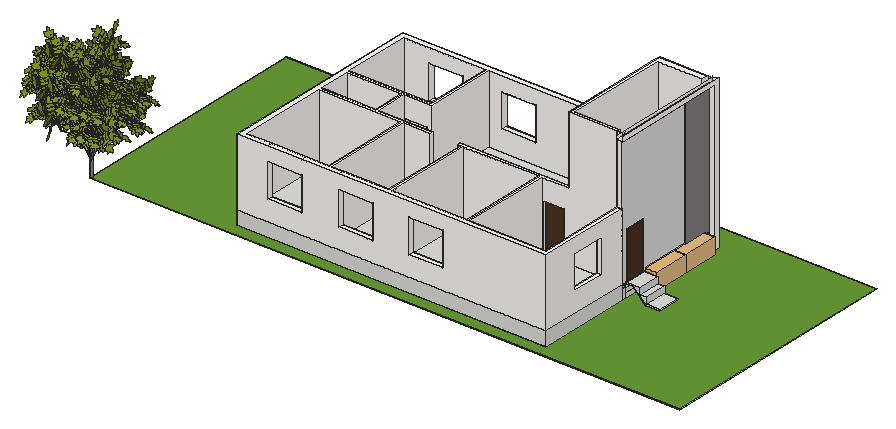
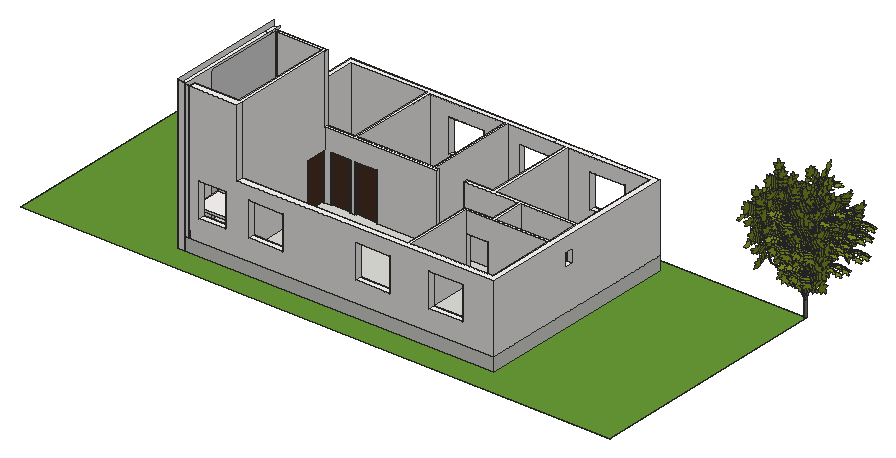
# SketchUp Ruby script. Lengths in inches.
U = 1.inch
M = Sketchup.active_model
def pt(a) = Geom::Point3d.new(a.map { |v| v * U })
def face(e, loops, mat)
  f = e.add_face(loops[0].map { |a| pt(a) })
  loops[1..].each { |l| e.add_face(l.map { |a| pt(a) }).erase! }
  f.material = f.back_material = mat if mat
  f
end
# faces: each face lists its corners as indices into pts; further lists are holes
def faces(e, pts, list, mat = nil) = list.each { |f| face(e, (f[0].is_a?(Array) ? f : [f]).map { |l| l.map { |i| pts[i] } }, mat) }
# xy, xz, yz: faces in a plane at the given z, y or x. An outline is a flat list of corners, or four numbers for a rectangle; further outlines are holes
def ring(l) = l.size == 4 ? [[l[0], l[1]], [l[2], l[1]], [l[2], l[3]], [l[0], l[3]]] : l.each_slice(2).to_a
def flat(e, list, mat, &to3) = list.each { |f| face(e, (f[0].is_a?(Array) ? f : [f]).map { |l| ring(l).map { |u, v| to3.(u, v) } }, mat) }
def xy(e, z, list, mat = nil) = flat(e, list, mat) { |x, y| [x, y, z] }
def xz(e, y, list, mat = nil) = flat(e, list, mat) { |x, z| [x, y, z] }
def yz(e, x, list, mat = nil) = flat(e, list, mat) { |y, z| [x, y, z] }
def lines(e, pts, list) = list.each { |a, b| e.add_line(pt(pts[a]), pt(pts[b])) }
# prism: a flat outline (further loops are holes) pulled along v
def prism(e, loops, v, mat = nil)
  f = face(e, loops, mat); d = Geom::Vector3d.new(v.map { |x| x * U })
  f.pushpull(f.normal.samedirection?(d) ? d.length : -d.length)
end
def box(e, o, s, mat = nil) = prism(e, [[o, [o[0] + s[0], o[1], o[2]], [o[0] + s[0], o[1] + s[1], o[2]], [o[0], o[1] + s[1], o[2]]]], [0, 0, s[2]], mat)
def at(x, y, z, deg = 0) = Geom::Transformation.translation(pt([x, y, z])) * Geom::Transformation.rotation(ORIGIN, Z_AXIS, deg.degrees)
def axes(o, x, y, z) = Geom::Transformation.new([*x, 0, *y, 0, *z, 0, *pt(o).to_a, 1])
def part(name) = M.definitions.add(name)
# library, detail: a bought-in or finely detailed component or shape, given as its bounding box
def library(name, o, s) = part(name).tap { |d| box(d.entities, o, s) }
def detail(e, o, s) = box(e.add_group.entities, o, s)
def put(e, d, t, mat = nil) = e.add_instance(d, t).tap { |i| i.material = mat if mat }
def group(e, t, mat = nil) = e.add_group.tap { |g| g.transformation = t; g.material = mat if mat }.entities
root = M.entities
M.materials.add("3D66_SU_1574822641685_001").color = [135, 150, 36]
M.materials.add("3D66_SU_1574822641883_002").color = [178, 165, 164]
M.materials.add("3D66_SU_1574822642012_003").color = [128, 125, 127]
M.materials.add("Polis06_194").color = [79, 50, 36]
M.materials.add("[0010_Snow]").color = [255, 250, 250]
M.materials.add("[Brick Tumbled]").color = [135, 132, 132]
M.materials.add("[Color M01]").color = [226, 226, 226]
M.materials.add("[Grass Dark Green]").color = [106, 157, 55]
c1 = part("Group16\#1")
prism(c1.entities,[[[640.68,60.08,-12.85],[640.68,60.08,-11.85],[640.68,36.46,-11.85],[640.68,36.46,-17.72],[640.68,24.64,-17.72],[640.68,24.64,-23.6],[640.68,1.02,-23.6],[640.68,1.02,-24.6],[640.68,24.88,-24.6],[640.68,48.5,-12.85]]],[-39.375,0,0])
c2 = part("Group7\#1")
p = [[645.1,1113.3,118],[645.1,1115.23,118],[645.1,1197.92,159.125],[645.1,1235.36,159.125],[723.92,1235.36,159.125],[723.92,1197.92,159.125],
  [723.92,1103.42,206.125],[723.92,1091.61,206.125],[680.6,1113.3,118],[680.6,1115.23,118],[680.6,1197.92,159.125],[680.6,1199.86,159.125],
  [688.42,1199.86,159.125],[688.42,1197.92,159.125],[688.42,1103.42,206.125],[688.42,1091.61,206.125]]
lines(c2.entities,p,[[0,1],[1,2],[2,3],[3,4],[4,5],[5,6],[6,7],[8,9],[9,10],[10,11],[11,12],[12,13],
  [13,14],[14,15]])
c3 = part("Group6\#1")
xy(c3.entities,114.0625,[[643.17,1127.05,682.54,1127.97]])
xy(c3.entities,118,[[643.17,1115.23,682.54,1127.05]])
xy(c3.entities,123.875,[[643.17,1127.05,682.54,1138.86]])
xy(c3.entities,129.75,[[643.17,1138.86,682.54,1150.67]])
xy(c3.entities,135.625,[[643.17,1150.67,682.54,1162.48]])
xy(c3.entities,141.5,[[643.17,1162.48,682.54,1174.3]])
xy(c3.entities,147.375,[[643.17,1174.3,682.54,1186.11]])
xy(c3.entities,153.25,[[643.17,1186.11,682.54,1197.92]])
xy(c3.entities,155.1875,[[686.48,1185.18,686.48,1197.92,682.54,1197.92,682.54,1210.66,643.17,1210.66,643.17,1237.3,725.85,1237.3,725.85,1185.18]])
xy(c3.entities,159.125,[[686.48,1186.11,725.85,1186.11,725.85,1237.3,643.17,1237.3,643.17,1197.92,686.48,1197.92]])
xy(c3.entities,165,[[686.48,1174.3,725.85,1186.11]])
xy(c3.entities,170.875,[[686.48,1162.48,725.85,1174.3]])
xy(c3.entities,176.75,[[686.48,1150.67,725.85,1162.48]])
xy(c3.entities,182.625,[[686.48,1138.86,725.85,1150.67]])
xy(c3.entities,188.5,[[686.48,1127.05,725.85,1138.86]])
xy(c3.entities,194.375,[[686.48,1115.23,725.85,1127.05]])
xy(c3.entities,200.25,[[686.48,1103.42,725.85,1115.23]])
xy(c3.entities,206.125,[[686.48,1091.61,725.85,1103.42]])
xz(c3.entities,1103.42,[[686.48,200.25,725.85,206.125]])
xz(c3.entities,1115.23,[[686.48,194.375,725.85,200.25]])
xz(c3.entities,1127.05,[[643.17,118,682.54,123.875],[686.48,188.5,725.85,194.375]])
xz(c3.entities,1138.86,[[643.17,123.875,682.54,129.75],[686.48,182.625,725.85,188.5]])
xz(c3.entities,1150.67,[[643.17,129.75,682.54,135.625],[686.48,176.75,725.85,182.625]])
xz(c3.entities,1162.48,[[643.17,135.625,682.54,141.5],[686.48,170.875,725.85,176.75]])
xz(c3.entities,1174.3,[[643.17,141.5,682.54,147.375],[686.48,165,725.85,170.875]])
xz(c3.entities,1186.11,[[643.17,147.375,682.54,153.25],[686.48,159.125,725.85,165]])
xz(c3.entities,1197.92,[[643.17,153.25,682.54,159.125],[682.54,155.1875,686.48,159.125]])
xz(c3.entities,1237.3,[[643.17,155.1875,725.85,159.125]])
yz(c3.entities,643.17,[[1127.05,114.0625,1127.05,123.875,1138.86,123.875,1138.86,129.75,1150.67,129.75,1150.67,135.625,1162.48,135.625,1162.48,141.5,1174.3,141.5,1174.3,147.375,1186.11,147.375,1186.11,153.25,1197.92,153.25,1197.92,159.125,1237.3,159.125,1237.3,155.1875,1210.66,155.1875,1127.97,114.0625]])
yz(c3.entities,682.54,[[1127.05,114.0625,1127.97,114.0625,1210.66,155.1875,1197.92,155.1875,1197.92,153.25,1186.11,153.25,1186.11,147.375,1174.3,147.375,1174.3,141.5,1162.48,141.5,1162.48,135.625,1150.67,135.625,1150.67,129.75,1138.86,129.75,1138.86,123.875,1127.05,123.875]])
yz(c3.entities,686.48,[[1185.18,155.1875,1090.68,202.1875,1091.61,202.1875,1091.61,206.125,1103.42,206.125,1103.42,200.25,1115.23,200.25,1115.23,194.375,1127.05,194.375,1127.05,188.5,1138.86,188.5,1138.86,182.625,1150.67,182.625,1150.67,176.75,1162.48,176.75,1162.48,170.875,1174.3,170.875,1174.3,165,1186.11,165,1186.11,159.125,1197.92,159.125,1197.92,155.1875]])
yz(c3.entities,725.85,[[1185.18,155.1875,1237.3,155.1875,1237.3,159.125,1186.11,159.125,1186.11,165,1174.3,165,1174.3,170.875,1162.48,170.875,1162.48,176.75,1150.67,176.75,1150.67,182.625,1138.86,182.625,1138.86,188.5,1127.05,188.5,1127.05,194.375,1115.23,194.375,1115.23,200.25,1103.42,200.25,1103.42,206.125,1091.61,206.125,1091.61,202.1875,1090.68,202.1875]])
p = [[643.17,1127.97,114.0625],[643.17,1210.66,155.1875],[682.54,1210.66,155.1875],[682.54,1127.97,114.0625],[725.85,1185.18,155.1875],[725.85,1090.68,202.1875],
  [686.48,1090.68,202.1875],[686.48,1185.18,155.1875]]
faces(c3.entities,p,[[0,1,2,3],[4,5,6,7]])
put(c3.entities,c2,at(0,0,39.375))
c4 = library("Group8",[-183.25,9.15,0],[25.91,56.79,43.93])
c5 = part("Group\#3")
xy(c5.entities,0,[[0,0,4.72,1.18],[0,34.25,4.72,35.43]],"Polis06_194")
xy(c5.entities,85.26,[[0,1.18,4.72,34.25]],"Polis06_194")
xy(c5.entities,86.61,[[0,0,4.72,35.43]],"Polis06_194")
xz(c5.entities,0,[[0,0,4.72,86.61]],"Polis06_194")
xz(c5.entities,1.18,[[0,0,2.36,85.26],[2.36,0,4.72,85.26]],"Polis06_194")
xz(c5.entities,34.25,[[0,0,4.72,85.26]],"Polis06_194")
xz(c5.entities,35.43,[[0,0,4.72,86.61]],"Polis06_194")
yz(c5.entities,0,[[0,0,1.18,86.61],[34.25,0,35.43,86.61],[1.18,85.26,34.25,86.61]],"Polis06_194")
yz(c5.entities,2.36,[[1.18,0,34.25,0,34.25,85.21,1.18,85.26]],"Polis06_194")
yz(c5.entities,4.72,[[0,0,1.18,86.61],[34.25,0,35.43,86.61],[1.18,85.26,34.25,86.61]],"Polis06_194")
c6 = part("rama-acacia")
p = [[-13.8,1.01,-1.08],[-13.61,0.91,-1.04],[-13.61,0.85,-1.06],[-14.07,0.85,-1.21],[-15.17,0.86,-1.58],[-15.95,0.92,-1.83],
  [-16.01,1,-1.83],[-16.01,1.17,-1.78],[-16.07,1.93,-1.6],[-16.4,2.73,-1.5],[-16.65,3.06,-1.5],[-17.13,4.01,-1.41],
  [-17.78,4.7,-1.44],[-18.28,5.07,-1.51],[-18.57,5.18,-1.58],[-18.91,5.47,-1.62],[-19.07,5.48,-1.67],[-19.35,5.61,-1.73],
  [-19.51,5.64,-1.78],[-19.38,5.57,-1.75],[-19.33,5.5,-1.75],[-19.31,5.23,-1.82],[-19.38,5.08,-1.89],[-19.41,4.84,-1.96],
  [-19.36,4.59,-2.01],[-19.43,4.55,-2.04],[-19.36,4.15,-2.125],[-19.21,3.7,-2.19],[-18.875,3.1,-2.24],[-18.61,2.78,-2.24],
  [-17.83,2.19,-2.13],[-17.4375,1.85,-2.09],[-17.04,1.49,-2.05],[-16.61,1.24,-1.97],[-16.17,1.0625,-1.87],[-16.06,0.95,-1.86],
  [-16.06,0.91,-1.87],[-16.32,0.9,-1.96],[-16.7,0.88,-2.1],[-17.05,0.91,-2.21],[-17.61,1.15,-2.33],[-18.06,1.29,-2.45],
  [-18.88,1.53,-2.67],[-20.25,1.46,-3.15],[-20.59,1.49,-3.26],[-20.79,1.37,-3.36],[-21.08,1.2,-3.5],[-21.28,1.22,-3.5625],
  [-21.48,0.94,-3.71],[-21.79,0.5,-3.93],[-22.02,0.17,-4.1],[-22.11,0.05,-4.16],[-22.21,-0.02,-4.21],[-22.375,-0.05,-4.28],
  [-22.375,-0.07,-4.28],[-22.18,-0.09,-4.22],[-22.11,-0.07,-4.19],[-21.78,-0.1,-4.09],[-21.6,-0.18,-4.05],[-21.52,-0.27,-4.04],
  [-21.33,-0.33,-4],[-20.94,-0.54,-3.92],[-20.6875,-0.63,-3.86],[-20.54,-0.68,-3.82],[-20.42,-0.67,-3.78],[-20.09,-0.46,-3.61],
  [-19.8,-0.24,-3.45],[-19.21,-0.02,-3.19],[-18.48,0.08,-2.92],[-17.72,0.38,-2.58],[-17.4,0.5,-2.4375],[-16.93,0.75,-2.21],
  [-16.78,0.8,-2.15],[-16.1,0.83,-1.91],[-16.0625,0.81,-1.9],[-16.08,0.77,-1.91],[-16.27,0.72,-1.99],[-16.88,0.39,-2.29],
  [-17.1875,0.15,-2.46],[-17.27,0.02,-2.52],[-17.94,-0.52,-2.89],[-17.94,-0.59,-2.91],[-18.08,-0.68,-2.99],[-18.13,-0.86,-3.05],
  [-18.56,-1.55,-3.38],[-18.71,-2.11,-3.58],[-18.79,-2.61,-3.74],[-18.86,-2.84,-3.83],[-18.87,-3.07,-3.89],[-18.84,-3.22,-3.92],
  [-18.8,-3.26,-3.92],[-18.76,-3.47,-3.96],[-18.76,-3.6,-4],[-18.67,-3.8,-4.02],[-18.61,-3.92,-4.04],[-18.58,-4.11,-4.07],
  [-18.53,-4.18,-4.08],[-18.58,-4.35,-4.14],[-18.65,-4.43,-4.18],[-18.72,-4.51,-4.23],[-18.8125,-4.51,-4.26],[-18.8125,-4.53,-4.26],
  [-18.72,-4.54,-4.24],[-18.66,-4.49,-4.21],[-18.58,-4.43,-4.16],[-18.35,-4.23,-4.03],[-18.32,-4.17,-4],[-18.22,-4.125,-3.95],
  [-18.1,-4,-3.88],[-17.79,-3.72,-3.7],[-17.68,-3.51,-3.61],[-17.32,-3.13,-3.38],[-17.24,-2.94,-3.31],[-16.78,-2.12,-2.93],
  [-16.48,-1.78,-2.73],[-16.3,-1.28,-2.54],[-16.05,-0.75,-2.3125],[-15.89,-0.2,-2.11],[-15.89,0.39,-1.95],[-15.96,0.79,-1.87],
  [-15.91,0.82,-1.84],[-15.27,0.8,-1.63],[-14.18,0.76,-1.27],[-13.78,0.73,-1.15],[-13.78,0.67,-1.16],[-14.23,0.54,-1.35],
  [-14.65,0.33,-1.55],[-14.97,0.02,-1.74],[-15.25,-0.36,-1.9375],[-15.57,-0.72,-2.14],[-15.96,-1.64,-2.52],[-16.2,-2.51,-2.84],
  [-16.2,-3.12,-3],[-16.14,-3.41,-3.06],[-16.1,-3.75,-3.14],[-16.1,-4.09,-3.23],[-16.2,-4.25,-3.3],[-16.2,-4.28,-3.3125],
  [-16.08,-4.19,-3.24],[-15.98,-4.08,-3.18],[-15.96,-3.94,-3.14],[-15.96,-3.8125,-3.1],[-15.9,-3.72,-3.06],[-15.68,-3.55,-2.9375],
  [-15.51,-3.49,-2.86],[-15.3,-3.33,-2.75],[-15.23,-3.17,-2.68],[-15.01,-3.03,-2.57],[-14.875,-2.83,-2.47],[-14.6,-2.59,-2.3125],
  [-14.4,-2.27,-2.16],[-14.12,-1.6,-1.89],[-13.91,-1.1,-1.68],[-13.67,-0.83,-1.53],[-13.53,-0.45,-1.38],[-13.53,0.67,-1.08],
  [-13.53,0.69,-1.07],[-13.38,0.86,-0.98],[-13.38,0.92,-0.96],[-13.32,1.03,-0.91],[-13.32,1.35,-0.82],[-13.28,1.49,-0.77],
  [-13.28,1.99,-0.64],[-13.44,2.67,-0.51],[-13.72,3.31,-0.43],[-13.93,3.71,-0.4],[-14.1,4.39,-0.27],[-14.5625,5.06,-0.25],
  [-14.89,5.62,-0.21],[-15.33,6.1,-0.23],[-15.65,6.8,-0.15],[-15.79,6.89,-0.18],[-15.61,6.52,-0.22],[-15.51,6.32,-0.24],
  [-15.45,6.28,-0.23],[-15.52,6,-0.32],[-15.63,5.6875,-0.45],[-15.77,4.97,-0.68],[-15.7,4.25,-0.85],[-15.46,3,-1.11],
  [-15,2.03,-1.21],[-14.3,1.29,-1.17],[-12.41,6.01,0.65],[-12.44,6.14,0.68],[-12.41,6.29,0.73],[-12.43,6.29,0.73],
  [-12.44,6.26,0.72],[-12.47,6.15,0.68],[-12.49,6.07,0.66],[-12.57,5.75,0.55],[-12.67,5.36,0.43],[-12.79,4.875,0.28],
  [-12.83,4.52,0.18],[-12.83,3.99,0.04],[-12.73,3.11,-0.18],[-12.58,2.52,-0.3125],[-12.3,1.97,-0.41],[-11.88,1.51,-0.46],
  [-11.37,1.0625,-0.48],[-10.75,0.75,-0.45],[-10.75,0.68,-0.47],[-12.55,0.7,-0.79],[-13.21,0.79,-0.89],[-13.2,0.67,-0.92],
  [-12.56,0.62,-0.82],[-11.15,0.56,-0.58],[-10.79,0.54,-0.52],[-10.72,0.52,-0.51],[-10.72,0.5,-0.52],[-10.87,0.47,-0.55],
  [-11.14,0.41,-0.62],[-11.39,0.27,-0.7],[-11.625,-0.01,-0.82],[-11.8,-0.43,-0.96],[-11.83,-0.57,-1],[-12.02,-1.08,-1.17],
  [-12.1,-1.39,-1.27],[-12.17,-1.95,-1.4375],[-12.17,-2.77,-1.65],[-12.09,-3.59,-1.86],[-11.86,-4.26,-2],[-11.8125,-4.4,-2.03],
  [-11.84,-4.49,-2.05],[-11.91,-4.6,-2.1],[-11.97,-4.65,-2.12],[-11.98,-4.67,-2.13],[-11.92,-4.65,-2.11],[-11.84,-4.59,-2.08],
  [-11.77,-4.52,-2.05],[-11.74,-4.47,-2.03],[-11.37,-4.3125,-1.92],[-10.95,-4.0625,-1.78],[-10.82,-3.89,-1.71],[-10.64,-3.57,-1.59],
  [-10.41,-3.05,-1.41],[-10.27,-2.73,-1.3],[-10.07,-1.88,-1.03],[-10.15,-0.71,-0.73],[-10.31,-0.1,-0.6],[-10.5,0.4,-0.5],
  [-10.5,0.48,-0.48],[-10.44,0.53,-0.45],[-10.39,0.64,-0.42],[-10.52,0.73,-0.42],[-10.44,0.93,-0.35],[-10.44,1.2,-0.28],
  [-10.32,1.47,-0.18],[-10.48,2.6875,0.12],[-10.43,2.96,0.2],[-10.75,3.87,0.38],[-11.26,4.93,0.57],[-11.8,5.54,0.64],
  [-12.37,5.93,0.64],[-7.78,0.19,-0.06],[-7.78,0.25,-0.04],[-7.75,0.39,0],[-7.89,0.4,-0.02],[-7.96,0.46,-0.02],
  [-7.96,0.49,-0.01],[-7.76,0.62,0.06],[-7.53,0.99,0.2],[-7.31,1.78,0.45],[-7.31,2.74,0.71],[-7.63,3.6875,0.9],
  [-8.02,4.57,1.07],[-8.66,5.23,1.13],[-8.83,5.4,1.14],[-8.92,5.54,1.16],[-9.1,5.64,1.16],[-9.08,5.6,1.15],
  [-9.02,5.56,1.15],[-8.94,5.46,1.14],[-8.9,5.37,1.12],[-8.9375,5.25,1.08],[-9.14,4.92,0.96],[-9.31,4.5625,0.83],
  [-9.39,3.73,0.6],[-9.44,2.76,0.32],[-9.23,1.59,0.05],[-8.82,0.9,-0.06],[-8.36,0.59,-0.0625],[-8.14,0.51,-0.04],
  [-8.05,0.48,-0.03],[-8.05,0.46,-0.04],[-8.12,0.43,-0.06],[-10.1,0.49,-0.4],[-8.22,0.3125,-0.11],[-8.22,0.25,-0.125],
  [-8.53,0.13,-0.21],[-8.8,-0.16,-0.34],[-8.96,-0.61,-0.49],[-8.96,-0.87,-0.56],[-9.16,-1.42,-0.74],[-9.13,-1.77,-0.83],
  [-9.09,-1.83,-0.84],[-9.125,-1.92,-0.87],[-9.125,-2.13,-0.93],[-9.08,-2.23,-0.95],[-9.15,-2.39,-1],[-9.11,-2.67,-1.07],
  [-9.03,-2.86,-1.11],[-9.07,-3.03,-1.16],[-8.97,-3.23,-1.19],[-8.93,-3.44,-1.24],[-8.93,-3.71,-1.32],[-8.79,-4.05,-1.38],
  [-8.7,-4.25,-1.42],[-8.7,-4.39,-1.46],[-8.76,-4.53,-1.5],[-8.77,-4.65,-1.54],[-8.64,-4.55,-1.49],[-8.27,-4.22,-1.33],
  [-8.1875,-4.06,-1.27],[-8.07,-3.98,-1.23],[-7.98,-3.79,-1.17],[-7.79,-3.59,-1.08],[-7.64,-3.3,-0.97],[-7.64,-3.25,-0.96],
  [-7.59,-3.21,-0.9375],[-7.52,-2.93,-0.85],[-7.52,-2.85,-0.83],[-7.47,-2.81,-0.81],[-7.3,-2.09,-0.59],[-7.32,-2.01,-0.57],
  [-7.27,-1.95,-0.54],[-7.1875,-1.57,-0.42],[-7.17,-1.46,-0.39],[-7.17,-1.16,-0.3125],[-7.23,-0.61,-0.17],[-7.49,-0.15,-0.1],
  [-13.39,-0.07,-1.23],[-13.39,0.25,-1.14],[-13.49,0.5625,-1.09],[-4.5625,0.33,0.09],[-4.22,0.49,0.13],[-4,0.7,0.1875],
  [-3.86,0.99,0.26],[-3.77,1.41,0.38],[-3.7,1.73,0.46],[-3.77,1.99,0.53],[-3.85,2.17,0.58],[-3.88,2.57,0.6875],
  [-3.98,2.9,0.78],[-4.0625,2.97,0.8],[-4.1,3.14,0.84],[-4.1875,3.25,0.87],[-4.27,3.55,0.95],[-4.31,3.71,0.99],
  [-4.42,3.9,1.04],[-4.625,4.2,1.125],[-4.72,4.39,1.18],[-4.89,4.57,1.23],[-4.98,4.73,1.27],[-5,4.72,1.26],
  [-5.01,4.51,1.21],[-4.96,4.32,1.16],[-4.97,4.27,1.14],[-5.14,3.78,1.01],[-5.3,3.39,0.91],[-5.44,2.76,0.74],
  [-5.5,2.09,0.56],[-5.57,1.78,0.48],[-5.57,1.42,0.38],[-5.57,1.09,0.29],[-5.47,0.72,0.19],[-5.22,0.44,0.12],
  [-4.93,0.27,0.07],[-4.76,0.22,0.06],[-4.76,0.18,0.05],[-4.83,0.16,0.04],[-5.26,0,0],[-5.34,-0.04,-0.01],
  [-5.47,-0.22,-0.06],[-5.51,-0.6,-0.16],[-5.42,-1.09,-0.29],[-5.28,-1.49,-0.4],[-5.21,-1.87,-0.5],[-5.11,-2.15,-0.57],
  [-5.08,-2.34,-0.63],[-5.01,-2.47,-0.66],[-4.96,-2.69,-0.72],[-4.86,-2.9375,-0.79],[-4.84,-3.07,-0.82],[-4.77,-3.18,-0.85],
  [-4.74,-3.43,-0.92],[-4.7,-3.71,-0.99],[-4.62,-3.89,-1.04],[-4.58,-3.98,-1.07],[-4.58,-3.83,-1.03],[-4.51,-3.67,-0.98],
  [-4.3,-3.32,-0.89],[-4.16,-3.09,-0.83],[-4.16,-2.98,-0.8],[-4.11,-2.92,-0.78],[-4.02,-2.8,-0.75],[-3.95,-2.59,-0.69],
  [-3.95,-2.33,-0.625],[-3.86,-2.26,-0.6],[-3.86,-2.02,-0.54],[-3.86,-1.44,-0.39],[-3.94,-1.22,-0.33],[-3.94,-1.08,-0.29],
  [-4,-0.96,-0.26],[-4,-0.87,-0.23],[-4.0625,-0.8125,-0.22],[-4.16,-0.54,-0.14],[-4.39,-0.24,-0.06],[-4.61,-0.08,-0.02],
  [-4.77,-0.03,-0.01],[-4.77,-0.01,0],[-4.65,-0.01,0],[-4.61,0.19,0.05],[-4.66,0.23,0.0625],[-4.63,0.29,0.08],
  [-4.07,0.17,0.04],[0,-0.24,-0.06],[0,0,0],[-0.5,0.04,0.01],[-1.58,0.08,0.02]]
faces(c6.entities,p,[[0,1,2,3,4,5,6,7,8,9,10,11,12,13,14,15,16,17,18,19,20,21,22,23,24,25,26,27,28,29,30,31,32,33,34,35,36,37,38,39,40,41,42,43,44,45,46,47,48,49,50,51,52,53,54,55,56,57,58,59,60,61,62,63,64,65,66,67,68,69,70,71,72,73,74,75,76,77,78,79,80,81,82,83,84,85,86,87,88,89,90,91,92,93,94,95,96,97,98,99,100,101,102,103,104,105,106,107,108,109,110,111,112,113,114,115,116,117,118,119,120,121,122,123,124,125,126,127,128,129,130,131,132,133,134,135,136,137,138,139,140,141,142,143,144,145,146,147,148,149,150,151,152,153,154,155,156,157,158,159,160,161,162,163,164,165,166,167,168,169,170,171,172,173,174,175,176,177,178,179,180,181],[182,183,184,185,186,187,188,189,190,191,192,193,194,195,196,197,198,199,200,201,202,203,204,205,206,207,208,209,210,211,212,213,214,215,216,217,218,219,220,221,222,223,224,225,226,227,228,229,230,231,232,233,234,235,236,237,238,239,240,241,242,243,244,245,246,247,248,249,250,251,252],[253,254,255,256,257,258,259,260,261,262,263,264,265,266,267,268,269,270,271,272,273,274,275,276,277,278,279,280,281,282,283,284,242,241,285,286,287,288,289,290,291,292,293,294,295,296,297,298,299,300,301,302,303,304,305,306,307,308,309,310,311,312,313,314,315,316,317,318,319,320,321,322,323,324,325,326,327,328,329],[154,330,331,332,155],[333,334,335,336,337,338,339,340,341,342,343,344,345,346,347,348,349,350,351,352,353,354,355,356,357,358,359,360,361,362,363,364,365,366,367,368,369,370,371,372,373,374,375,376,377,378,379,380,381,382,383,384,385,386,387,388,389,390,391,392,393,394,395,396,397,398,399,400,401,402,403,404,405,406,407,408,409,410,411,412,413],[156,203,157],[202,157,203],[414,411,410,415,416,417,418],
  [254,370,255],[369,255,370]],"3D66_SU_1574822641685_001")
c7 = part("ramas")
put(c7.entities,c6,axes([0.11,0.06,-0.22],[-0.42655,-0.79206,-0.43668],[0.22445,0.37501,-0.89944],[0.87617,-0.48167,0.01782]))
put(c7.entities,c6,axes([0.14,0.21,0.02],[0.24321,-0.08852,-0.96593],[0.34202,0.93969,0],[0.90767,-0.33037,0.25882]))
put(c7.entities,c6,at(0,0.24,0.06))
put(c7.entities,c6,axes([0.11,0.45,0.57],[-0.42655,0.68302,0.5929],[0.22445,-0.55509,0.80093],[0.87617,0.47472,0.08347]))
put(c7.entities,c6,axes([0.11,0.73,0.01],[-0.42655,0.88928,-0.16503],[0.22445,0.28083,0.93314],[0.87617,0.36099,-0.31939]))
c8 = part("rama principal")
put(c8.entities,c6,axes([-20.25,-0.15,12.84],[0.38818,-0.89018,-0.23852],[0.89018,0.42916,-0.15296],[0.23852,-0.15296,0.95902]))
put(c8.entities,c6,at(-20.48,0,12.88))
put(c8.entities,c6,axes([-20.6875,-0.1,12.85],[0.57358,0.79124,0.21201],[-0.79124,0.60214,-0.10661],[-0.21201,-0.10661,0.97144]))
put(c8.entities,c6,axes([-20.375,-0.01,13.02],[-0.37792,0.77975,-0.49916],[-0.65887,0.15226,0.73669],[0.65043,0.60729,0.45621]))
put(c8.entities,c6,axes([-20.34,-0.04,12.83],[0.24321,-0.08852,-0.96593],[0.34202,0.93969,0],[0.90767,-0.33037,0.25882]))
put(c8.entities,c6,axes([-20.375,-0.18,12.6],[-0.42655,-0.79206,-0.43668],[0.22445,0.37501,-0.89944],[0.87617,-0.48167,0.01782]))
put(c8.entities,c7,at(-11.43,0,7.77))
g1 = group(c8.entities,at(0,0.2,0),"3D66_SU_1574822641883_002")
xz(g1,0.1,[[-0.15,-0.08,-3.26,5.59,-11.5,7.61,-18.23,12.71,-20.48,12.71,-20.48,13.05,-18.11,13.05,-11.35,7.92,-3.03,5.89,0.15,0.08]])
yz(g1,-20.48,[[0.1,12.71,-0.2,12.88,0.1,13.05]])
p = [[-0.15,0.1,-0.08],[0,-0.2,0],[-3.15,-0.2,5.74],[-3.26,0.1,5.59],[0.15,0.1,0.08],[-3.03,0.1,5.89],
  [-11.43,-0.2,7.77],[-11.5,0.1,7.61],[-11.35,0.1,7.92],[-18.17,-0.2,12.88],[-18.23,0.1,12.71],[-18.11,0.1,13.05],
  [-20.48,-0.2,12.88],[-20.48,0.1,12.71],[-20.48,0.1,13.05]]
faces(g1,p,[[0,1,2,3],[0,4,1],[1,4,5,2],[3,2,6,7],[2,5,8,6],[7,6,9,10],[6,8,11,9],[10,9,12,13],
  [9,11,14,12]])
c9 = part("Component\#1")
p = [[44.23,0.79,16.51],[35.57,0.79,41.625],[19.17,0.79,51.61],[7.37,0.79,32.7],[0.16,0.79,57.85],[31.31,0.79,23.98]]
lines(c9.entities,p,[[0,1],[1,2],[3,4],[5,3]])
g2 = group(c9.entities,at(44.23,0.79,-28.39))
xz(g2,0.2,[[-0.32,44.79,-8.95,69.78,-25.24,79.7,-24.89,80.28,-8.38,70.24,0.32,45.01]],"3D66_SU_1574822642012_003")
p = [[-0.32,0.2,44.79],[0,-0.39,44.9],[-8.67,-0.39,70.01],[-8.95,0.2,69.78],[0.32,0.2,45.01],[-8.38,0.2,70.24],
  [-25.06,-0.39,79.99],[-25.24,0.2,79.7],[-24.89,0.2,80.28]]
faces(g2,p,[[0,1,2,3],[0,4,1],[1,4,5,2],[3,2,6,7],[2,5,8,6],[8,7,6]],"3D66_SU_1574822642012_003")
g3 = group(c9.entities,at(44.23,0.79,-28.39),"3D66_SU_1574822642012_003")
p = [[-0.6,0.39,28.39],[0,-0.79,28.71],[-12.89,-0.52,52.37],[-13.25,0.19,52.17],[0.6,0.39,29.04],[-12.53,0.19,52.57]]
faces(g3,p,[[0,1,2,3],[4,0,3,5],[1,4,5,2]],"3D66_SU_1574822642012_003")
faces(g3,p,[[0,4,1],[5,3,2]])
g4 = group(c9.entities,at(44.23,0.79,-28.39))
prism(g4,[[[-37.03,0.1,61.04],[-36.7,0.1,61.13],[-36.86,-0.2,61.08]]],[-7.21,0,25.15],"3D66_SU_1574822642012_003")
g5 = group(c9.entities,at(44.23,0.79,-28.39))
prism(g5,[[[-13.04,0.2,52.05],[-12.81,0.2,52.69],[-12.92,-0.39,52.37]]],[-23.94,0,8.71],"3D66_SU_1574822642012_003")
c10 = part("Group\#7")
p = [[74.89,60.42,11.53],[61.97,60.42,35.1875]]
lines(c10.entities,p,[[0,1]])
put(c10.entities,c8,at(68.97,49.02,23.76))
put(c10.entities,c8,at(53.09,47.85,77.85))
put(c10.entities,c8,at(71.03,52.76,41.54))
put(c10.entities,c9,at(57.21,20.01,0,65))
put(c10.entities,c9,at(36.98,37.62,26.03,30))
put(c10.entities,c8,at(64.15,37.99,51.46))
put(c10.entities,c8,at(56.21,20.74,57.94))
put(c10.entities,c8,at(58.92,27.24,32.75))
put(c10.entities,c8,at(63.69,53.97,50.16))
put(c10.entities,c8,at(67.38,56.1,67.8))
put(c10.entities,c8,at(42.86,42.51,58.92))
xy(root,-24.1,[[96.82,90.85,1120.4,472.81]])
xy(root,-23.6,[[96.82,90.85,1120.4,518.11]],"[Grass Dark Green]")
xz(root,90.85,[[96.82,-24.1,1120.4,-23.6]])
yz(root,96.82,[[90.85,-24.1,90.85,-23.6,518.11,-23.6,472.81,-24.1]])
yz(root,1120.4,[[90.85,-24.1,472.81,-24.1,518.11,-23.6,90.85,-23.6]])
p = [[96.82,518.11,-23.6],[1120.4,518.11,-23.6],[1120.4,472.81,-24.1],[96.82,472.81,-24.1],[871.06,465.59,231.94],[871.06,465.59,-23.6],
  [871.06,285.7,0],[871.06,285.7,-26.4375],[871.06,278.08,118],[871.06,278.08,-23.6]]
faces(root,p,[[0,1,2,3]])
lines(root,p,[[4,5],[6,7],[8,9]])
g6 = group(root,at(98.11,92.93,-24.1),"3D66_SU_1574822642012_003")
xy(g6,0,[[-1.29,-2.08,-1.29,2.08,2.58,0]])
xy(g6,48.23,[[-1.02,-1.79,2.31,0,-1.02,1.79]])
p = [[2.58,0,0],[2.31,0,48.23],[-1.02,-1.79,48.23],[-1.29,-2.08,0],[-1.02,1.79,48.23],[-1.29,2.08,0]]
faces(g6,p,[[0,1,2,3],[2,4,5,3],[5,4,1,0]])
g7 = group(root,at(334.375,113.59,-23.6))
xy(g7,0,[[0,0,536.68,359.22]])
xy(g7,23.6,[[0,0,536.68,359.22]])
xz(g7,0,[[0,0,536.68,23.6]])
xz(g7,359.22,[[0,0,536.68,23.6]])
yz(g7,0,[[0,0,359.22,23.6]])
yz(g7,536.68,[[0,0,172.12,23.6],[172.12,0,212.49,23.6],[212.49,0,359.22,23.6]])
p = [[536.68,212.49,15.73],[536.68,172.14,15.73],[536.68,212.49,7.87],[536.68,172.125,7.87]]
lines(g7,p,[[0,1],[2,3]])
put(g7,c1,axes([596.77,-428.2,45.53],[0,1,0],[-1,0,0],[0,0,1.85098]))
g8 = group(root,at(334.375,113.59,0),"[0010_Snow]")
xy(g8,-23.6,[[536.68,352,548.48,360]])
xy(g8,0,[[0,0,0,360,528.14,360,528.14,349.125,450.875,349.125,450.875,208.61,445.13,208.61,445.13,349.125,157.8,349.125,157.8,225.1875,150.33,225.1875,150.33,230.78,152.05,230.78,152.05,349.125,10.58,349.125,10.58,230.78,113.11,230.78,113.11,225.1875,110.03,225.1875,110.03,201.57,104.59,201.57,104.59,225.1875,10.58,225.1875,10.58,170.33,104.59,170.33,104.59,171.88,110.03,171.88,110.03,170.33,113.76,170.33,113.76,164.2,10.58,164.2,10.58,9.4375,152.05,9.4375,152.05,164.2,150.07,164.2,150.07,170.33,203.14,170.33,203.14,164.2,157.72,164.2,157.72,9.4375,256.35,9.4375,256.35,164.49,251.29,164.49,251.29,170.33,354.04,170.33,354.04,164.49,261.37,164.49,261.37,9.4375,392.31,9.4375,392.31,170.33,400.41,170.33,400.41,164.49,397.5,164.49,397.5,9.4375,528.5,9.4375,528.5,164.49,536.68,164.49,536.68,0],[435.46,164.49,528.5,170.33]])
xy(g8,0,[[536.68,301.66,537.68,349.125],[528.14,349.125,536.68,352],[536.68,349.125,537.68,352]],"[Color M01]")
xy(g8,35.43,[[52.96,0,113.1,9.4375],[176.51,0,235.97,9.4375],[298.47,0,358.21,9.4375],[528.5,60.51,536.68,120.22],[54.3,349.125,113.03,360],
  [180.36,349.125,239.71,360],[365.54,349.125,424.86,360],[465.84,349.125,512.28,360]])
xy(g8,70.8,[[0,189.26,10.58,206.83]])
xy(g8,82.6,[[113.76,164.2,150.07,170.33],[354.04,164.49,392.31,170.33],[400.41,164.49,435.46,170.33],[445.13,170.33,450.875,208.61],[104.59,171.88,110.03,201.57],
  [113.11,225.1875,150.33,230.78]])
xy(g8,94.4,[[0,189.26,10.58,206.83]])
xy(g8,94.43,[[52.96,0,113.1,9.4375],[176.51,0,235.97,9.4375],[298.47,0,358.21,9.4375],[528.5,60.51,536.68,120.22],[54.3,349.125,113.03,360],
  [180.36,349.125,239.71,360],[365.54,349.125,424.86,360],[465.84,349.125,512.28,360]])
xy(g8,118,[[[0,0,52.96,0,52.96,9.4375,10.58,9.4375,10.58,164.2,152.05,164.2,152.05,9.4375,113.1,9.4375,113.1,0,176.51,0,176.51,9.4375,157.72,9.4375,157.72,164.2,203.14,164.2,203.14,170.33,110.03,170.33,110.03,225.1875,157.8,225.1875,157.8,349.125,445.13,349.125,445.13,360,0,360],[10.58,230.78,152.05,349.125],[10.58,170.33,104.59,225.1875]],[52.96,0,113.1,9.4375],[[176.51,0,536.68,0,536.68,164.49,528.5,164.49,528.5,9.4375,397.5,9.4375,397.5,164.49,445.13,164.49,445.13,170.33,251.29,170.33,251.29,164.49,256.35,164.49,256.35,9.4375,176.51,9.4375],[261.37,9.4375,392.31,164.49]]])
xy(g8,231.94,[[536.68,152.6875,548.48,172.49],[536.68,172.49,536.68,301.66,537.68,301.66,537.68,352,548.48,352,548.48,172.49]])
xy(g8,236,[[445.13,164.49,528.5,164.49,528.5,170.33,450.875,170.33,450.875,349.125,528.14,349.125,528.5,360,445.13,360]])
xz(g8,0,[[[0,0,536.68,118],[52.96,35.43,113.1,94.43],[298.47,35.43,358.21,94.43],[176.51,35.43,235.97,94.43]]])
xz(g8,9.4375,[[[10.58,0,152.05,118],[52.96,35.43,113.1,94.43]],[[157.72,0,256.35,118],[176.51,35.43,235.97,94.43]],[[261.37,0,392.31,118],[298.47,35.43,358.21,94.43]],[397.5,0,528.5,118]])
xz(g8,60.51,[[528.5,35.43,536.68,94.43]])
xz(g8,120.22,[[528.5,35.43,536.68,94.43]])
xz(g8,164.2,[[10.58,0,113.76,0,113.76,82.6,150.07,82.6,150.07,0,152.05,0,152.05,118,10.58,118],[157.72,0,203.14,118]])
xz(g8,164.49,[[251.29,0,256.35,118],[261.37,0,354.04,0,354.04,82.6,392.31,82.6,392.31,118,261.37,118],[397.5,0,400.41,0,400.41,82.6,435.46,82.6,435.46,0,528.5,0,528.5,236,445.13,236,445.13,118,397.5,118],[528.5,0,536.68,118],[528.5,118,536.68,236]])
xz(g8,170.33,[[10.58,0,104.59,118],[110.03,0,110.03,118,203.14,118,203.14,0,150.07,0,150.07,82.6,113.76,82.6,113.76,0],[251.29,0,251.29,118,445.13,118,445.13,82.6,450.875,82.6,450.875,0,435.46,0,435.46,82.6,400.41,82.6,400.41,0,392.31,0,392.31,82.6,354.04,82.6,354.04,0],[450.875,0,528.5,236]])
xz(g8,171.88,[[104.59,0,110.03,82.6]])
xz(g8,189.26,[[0,70.8,10.58,94.4]])
xz(g8,201.57,[[104.59,0,110.03,82.6]])
xz(g8,206.83,[[0,70.8,10.58,94.4]])
xz(g8,208.61,[[445.13,0,450.875,82.6]])
xz(g8,225.1875,[[10.58,0,104.59,118],[110.03,0,113.11,0,113.11,82.6,150.33,82.6,150.33,0,157.8,0,157.8,118,110.03,118]])
xz(g8,230.78,[[10.58,0,10.58,118,152.05,118,152.05,0,150.33,0,150.33,82.6,113.11,82.6,113.11,0]])
xz(g8,301.66,[[536.68,0,537.68,231.94]],"[Color M01]")
xz(g8,349.125,[[[10.58,0,152.05,118],[54.3,35.43,113.03,94.43]],[[157.8,0,445.13,118],[180.36,35.43,239.71,94.43],[365.54,35.43,424.86,94.43]],[[450.875,0,528.14,236],[465.84,35.43,512.28,94.43]]])
xz(g8,352,[[536.68,-23.6,548.48,-23.6,548.48,231.94,537.68,231.94,537.68,0,536.68,0]])
xz(g8,360,[[536.68,-23.6,536.68,236,548.48,239.94,548.48,-23.6],[528.5,-0.75,528.14,0,528.5,0],[528.5,-0.75,536.68,236],[[0,0,0,118,445.13,118,445.13,236,528.5,236,528.5,0],[180.36,35.43,239.71,94.43],[365.54,35.43,424.86,94.43],[54.3,35.43,113.03,94.43],[465.84,35.43,512.28,94.43]]])
yz(g8,0,[[[0,0,360,118],[189.26,70.8,206.83,94.4]]])
yz(g8,10.58,[[9.4375,0,164.2,118],[[170.33,0,225.1875,118],[189.26,70.8,206.83,94.4]],[230.78,0,349.125,118]])
yz(g8,52.96,[[0,35.43,9.4375,94.43]])
yz(g8,54.3,[[349.125,35.43,360,94.43]])
yz(g8,104.59,[[170.33,0,170.33,118,225.1875,118,225.1875,0,201.57,0,201.57,82.6,171.88,82.6,171.88,0]])
yz(g8,110.03,[[170.33,0,171.88,0,171.88,82.6,201.57,82.6,201.57,0,225.1875,0,225.1875,118,170.33,118]])
yz(g8,113.03,[[349.125,35.43,360,94.43]])
yz(g8,113.1,[[0,35.43,9.4375,94.43]])
yz(g8,113.11,[[225.1875,0,230.78,82.6]])
yz(g8,113.76,[[164.2,0,170.33,82.6]])
yz(g8,150.07,[[164.2,0,170.33,82.6]])
yz(g8,150.33,[[225.1875,0,230.78,82.6]])
yz(g8,152.05,[[9.4375,0,164.2,118],[230.78,0,349.125,118]])
yz(g8,157.72,[[9.4375,0,164.2,118]])
yz(g8,157.8,[[225.1875,0,349.125,118]])
yz(g8,176.51,[[0,35.43,9.4375,94.43]])
yz(g8,180.36,[[349.125,35.43,360,94.43]])
yz(g8,203.14,[[164.2,0,170.33,118]])
yz(g8,235.97,[[0,35.43,9.4375,94.43]])
yz(g8,239.71,[[349.125,35.43,360,94.43]])
yz(g8,251.29,[[164.49,0,170.33,118]])
yz(g8,256.35,[[9.4375,0,164.49,118]])
yz(g8,261.37,[[9.4375,0,164.49,118]])
yz(g8,298.47,[[0,35.43,9.4375,94.43]])
yz(g8,354.04,[[164.49,0,170.33,82.6]])
yz(g8,358.21,[[0,35.43,9.4375,94.43]])
yz(g8,365.54,[[349.125,35.43,360,94.43]])
yz(g8,392.31,[[9.4375,0,9.4375,118,164.49,118,164.49,82.6,170.33,82.6,170.33,0]])
yz(g8,397.5,[[9.4375,0,164.49,118]])
yz(g8,400.41,[[164.49,0,170.33,82.6]])
yz(g8,424.86,[[349.125,35.43,360,94.43]])
yz(g8,435.46,[[164.49,0,170.33,82.6]])
yz(g8,445.13,[[208.61,0,208.61,82.6,170.33,82.6,170.33,236,349.125,236,349.125,0],[164.49,118,170.33,236],[349.125,118,360,236]])
yz(g8,450.875,[[208.61,0,349.125,0,349.125,236,170.33,236,170.33,82.6,208.61,82.6]])
yz(g8,465.84,[[349.125,35.43,360,94.43]])
yz(g8,512.28,[[349.125,35.43,360,94.43]])
yz(g8,528.14,[[349.125,0,360,0,349.125,118]])
yz(g8,528.5,[[[9.4375,0,164.49,118],[60.51,35.43,120.22,94.43]],[164.49,0,170.33,236]])
yz(g8,536.68,[[164.49,-23.6,172.12,0],[172.12,-23.6,172.15,0,172.12,0],[301.66,-23.6,352,0],[352,-23.6,360,0],[[0,0,164.49,118],[60.51,35.43,120.22,94.43]],
  [301.66,0,301.66,231.94,170.33,231.94,170.33,236,360,236,360,0],[172.12,0,172.15,0,172.15,2.67],[152.6875,231.94,164.49,236],[164.49,231.94,170.33,236]])
yz(g8,536.68,[[164.49,0,164.49,231.94,301.66,231.94,301.66,0,212.49,0,212.49,82.6,173.3,82.6,172.15,2.67,172.12,0]],"[Color M01]")
yz(g8,537.68,[[301.66,0,352,231.94]],"[Brick Tumbled]")
yz(g8,548.48,[[352,-23.6,360,-23.6,360,239.94,152.6875,239.94,152.6875,231.94,352,231.94]])
p = [[528.5,360,-0.75],[528.14,349.125,118],[528.14,360,0],[528.5,360,0],[528.5,360,236],[528.14,349.125,236],
  [256.35,164.58,0],[256.35,164.49,0],[261.37,164.49,0],[261.37,164.58,0],[536.68,212.49,0],[536.68,172.15,0],
  [536.68,360,239.94],[536.68,360,236]]
faces(g8,p,[[0,1,2],[1,0,3,4,5]])
lines(g8,p,[[6,7],[8,9],[10,11],[12,13]])
put(g8,c3,at(-178.6,-899.1875,-114.0625,0.881))
put(root,c4,axes([1016.47,400.96,-23.6],[0.79351,0,0],[0,-1.10365,0],[0,0,0.6372]))
put(root,c4,axes([1016.47,464.34,-23.6],[0.79351,0,0],[0,-1.10365,0],[0,0,0.6372]))
put(root,c5,axes([780.52,282.39,0],[1,0,0],[0,1.12351,0],[0,0,0.95365]))
put(root,c5,axes([448.13,283.91,0],[-0.03128,-0.59692,0],[1.02201,-0.05356,0],[0,0,0.95365]))
put(root,c5,axes([688.41,283.91,0],[-0.03015,-0.57528,0],[1.07707,-0.05645,0],[0,0,0.95365]))
put(root,c5,axes([734.79,283.91,0],[-0.03202,-0.61095,0],[0.98632,-0.05169,0],[0,0,0.95365]))
put(root,c5,axes([439.68,285.47,0],[1,0,0],[0,0.83788,0],[0,0,0.95365]))
put(root,c5,axes([866.33,286.26,0],[1,0,0],[0,1.12351,0],[0,0,0.95365]))
put(root,c10,axes([30.75,192.16,4.76],[-0.15043,-1.21193,0],[1.30133,-0.1401,0],[0,0,1.6799]))
put(root,c10,axes([0,19.22,4.76],[1.31,0,0],[0,1.22,0],[0,0,1.6799]))
put(root,c10,axes([222.64,111.08,4.76],[-1.13449,0.61,0],[-0.655,-1.05655,0],[0,0,1.6799]))
put(root,c10,axes([168.4,-4.51,4.76],[0.11417,1.21536,0],[-1.30502,0.10633,0],[0,0,1.6799]))
